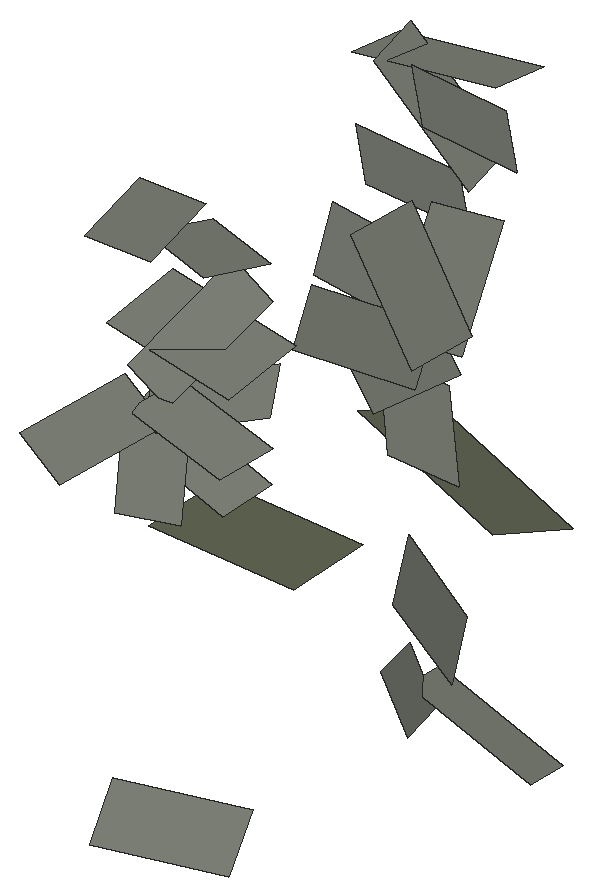
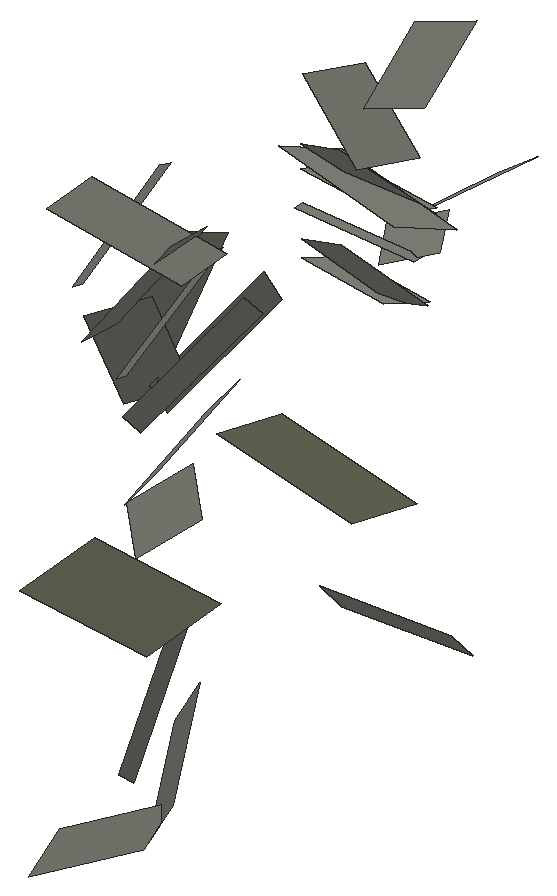
# SketchUp Ruby script. Lengths in inches.
U = 1.inch
M = Sketchup.active_model
def pt(a) = Geom::Point3d.new(a.map { |v| v * U })
def face(e, loops, mat)
  f = e.add_face(loops[0].map { |a| pt(a) })
  loops[1..].each { |l| e.add_face(l.map { |a| pt(a) }).erase! }
  f.material = f.back_material = mat if mat
  f
end
# faces: each face lists its corners as indices into pts; further lists are holes
def faces(e, pts, list, mat = nil) = list.each { |f| face(e, (f[0].is_a?(Array) ? f : [f]).map { |l| l.map { |i| pts[i] } }, mat) }
# xy, xz, yz: faces in a plane at the given z, y or x. An outline is a flat list of corners, or four numbers for a rectangle; further outlines are holes
def ring(l) = l.size == 4 ? [[l[0], l[1]], [l[2], l[1]], [l[2], l[3]], [l[0], l[3]]] : l.each_slice(2).to_a
def flat(e, list, mat, &to3) = list.each { |f| face(e, (f[0].is_a?(Array) ? f : [f]).map { |l| ring(l).map { |u, v| to3.(u, v) } }, mat) }
def xy(e, z, list, mat = nil) = flat(e, list, mat) { |x, y| [x, y, z] }
def xz(e, y, list, mat = nil) = flat(e, list, mat) { |x, z| [x, y, z] }
def yz(e, x, list, mat = nil) = flat(e, list, mat) { |y, z| [x, y, z] }
def lines(e, pts, list) = list.each { |a, b| e.add_line(pt(pts[a]), pt(pts[b])) }
# prism: a flat outline (further loops are holes) pulled along v
def prism(e, loops, v, mat = nil)
  f = face(e, loops, mat); d = Geom::Vector3d.new(v.map { |x| x * U })
  f.pushpull(f.normal.samedirection?(d) ? d.length : -d.length)
end
def box(e, o, s, mat = nil) = prism(e, [[o, [o[0] + s[0], o[1], o[2]], [o[0] + s[0], o[1] + s[1], o[2]], [o[0], o[1] + s[1], o[2]]]], [0, 0, s[2]], mat)
def at(x, y, z, deg = 0) = Geom::Transformation.translation(pt([x, y, z])) * Geom::Transformation.rotation(ORIGIN, Z_AXIS, deg.degrees)
def axes(o, x, y, z) = Geom::Transformation.new([*x, 0, *y, 0, *z, 0, *pt(o).to_a, 1])
def part(name) = M.definitions.add(name)
# library, detail: a bought-in or finely detailed component or shape, given as its bounding box
def library(name, o, s) = part(name).tap { |d| box(d.entities, o, s) }
def detail(e, o, s) = box(e.add_group.entities, o, s)
def put(e, d, t, mat = nil) = e.add_instance(d, t).tap { |i| i.material = mat if mat }
def group(e, t, mat = nil) = e.add_group.tap { |g| g.transformation = t; g.material = mat if mat }.entities
root = M.entities
M.materials.add("viburnumblaasdfas0df1w06d").color = [98, 102, 84]
M.materials.add("viburnumbladsadfasdfad0w122").color = [125, 129, 119]
c1 = part("Component\#315")
p = [[0.25,0,0],[2.05,0.01,0.35],[1.81,4.2,1.66],[0,4.19,1.3125]]
faces(c1.entities,p,[[0,1,2,3]],"viburnumbladsadfasdfad0w122")
c2 = part("viburnumblad2")
put(c2.entities,c1,axes([-19.23,-4.49,-32.18],[83.35428,0,0],[0,79.38502,0],[0,0,83.35428]))
c3 = part("Component\#314")
p = [[0.14,0,0],[2.58,0.05,0.25],[2.44,5.11,2.64],[0,5.05,2.39]]
faces(c3.entities,p,[[0,1,2,3]],"viburnumblaasdfas0df1w06d")
c4 = part("viburnumblad1\#2")
put(c4.entities,c3,axes([-37.25,6.23,19.31],[75.98784,0,0],[0,65.50676,0],[0,0,75.98784]))
put(root,c2,axes([1241.59,200.74,28.69],[-0.01126,-0.00309,0.00036],[0.00297,-0.01108,-0.00222],[0.00093,-0.00205,0.01147]))
put(root,c2,axes([1240.14,199.86,22.73],[0.01011,-0.00136,-0.00516],[0.0034,0.00814,0.00428],[0.00337,-0.00599,0.00744]))
put(root,c2,axes([1243,209.77,25.51],[-0.00283,0.01146,0.00038],[-0.0094,-0.00257,0.00741],[0.00704,0.00146,0.00821]))
put(root,c2,axes([1242.51,198.01,23.72],[-0.00968,0.00131,0.00494],[-0.00285,-0.01022,-0.00281],[0.00419,-0.00363,0.00837]))
put(root,c4,axes([1238.92,204.09,17.79],[-0.00228,-0.0125,-0.00287],[0.01428,-0.00152,-0.00471],[0.00336,-0.00314,0.01093]))
put(root,c2,axes([1242.72,210.15,24.1],[-0.00853,0.00601,0.00433],[-0.00446,-0.01051,0.00545],[0.00645,0.00235,0.00846]))
put(root,c2,axes([1243.16,208.5,21.67],[-0.00501,0.0098,0.00679],[-0.00808,-0.00821,0.00589],[0.00877,-0.00196,0.0093]))
put(root,c2,axes([1239.68,211.03,28.49],[-0.00073,-0.01199,-0.00108],[0.01339,-0.00063,-0.00213],[0.0019,-0.00123,0.01236]))
put(root,c2,axes([1240.09,198.93,12.3],[0.00083,-0.00664,-0.00958],[0.01085,0.00394,-0.00179],[0.00425,-0.00877,0.00644]))
put(root,c2,axes([1241.86,210.07,10.17],[-0.00779,-0.00011,0.00854],[0.00262,-0.01208,0.00224],[0.0089,0.00345,0.00816]))
put(root,c2,axes([1242.76,209.72,20.15],[-0.00997,0.00134,0.00814],[-0.00176,-0.01174,-0.00023],[0.00802,-0.0014,0.01005]))
put(root,c2,axes([1240.92,201.87,27.55],[-0.00596,-0.00978,-0.00229],[0.01005,-0.00579,-0.00143],[0.00006,-0.0027,0.01137]))
put(root,c2,axes([1240.07,201.3,25.98],[-0.00385,-0.0119,-0.00772],[0.01402,-0.00199,-0.00394],[0.00214,-0.0084,0.01187]))
put(root,c2,axes([1241.78,210.5,19.18],[-0.00949,-0.00826,0.00492],[0.00532,-0.00908,-0.00498],[0.00706,-0.00173,0.0107]))
put(root,c2,axes([1240.91,198.53,24.71],[0.00968,-0.00131,-0.00494],[0.00378,0.00904,0.00475],[0.00337,-0.00599,0.00744]))
put(root,c2,axes([1242.85,209.46,11.4],[-0.00627,0.00896,0.00619],[-0.00305,-0.00837,0.00903],[0.01046,0.00298,0.00629]))
put(root,c2,axes([1242.19,199.42,23.07],[-0.0092,-0.00594,0.0008],[0.00497,-0.0084,-0.00522],[0.00323,-0.00386,0.00866]))
put(root,c4,axes([1239.6,211.76,17],[-0.00406,-0.01328,0.00293],[0.01275,-0.00581,-0.00863],[0.008,0.00014,0.01172]))
put(root,c2,axes([1240.8125,199.62,23.74],[0.00449,-0.00779,-0.00619],[0.00881,0.00487,0.00016],[0.00266,-0.00553,0.00801]))
put(root,c2,axes([1241.22,200.35,22.63],[-0.00331,-0.00841,-0.00433],[0.01007,-0.00189,-0.00393],[0.00222,-0.00567,0.00805]))
put(root,c2,axes([1243.68,206.72,21.22],[-0.00309,0.00736,0.0079],[-0.00654,-0.00921,0.0057],[0.00929,-0.00262,0.00521]))
put(root,c2,axes([1241.17,211.13,10.67],[0.00148,-0.01296,0.00142],[0.00776,-0.00002,-0.00823],[0.00903,0.00196,0.00851]))
put(root,c2,axes([1244.27,210.09,26.35],[-0.00889,0.00626,0.00451],[-0.00413,-0.00973,0.00504],[0.00645,0.00235,0.00846]))
put(root,c2,axes([1242.8125,206.79,22.42],[0.00746,0.0085,-0.0048],[-0.00195,0.00645,0.00799],[0.00881,-0.00455,0.00477]))
put(root,c2,axes([1242.15,199.1,24.48],[-0.00334,-0.0097,-0.00381],[0.01007,-0.00189,-0.00393],[0.0026,-0.00465,0.00851]))
put(root,c2,axes([1244.22,205.89,22.33],[0.00278,0.01118,0.00257],[-0.00655,-0.00082,0.0102],[0.00931,-0.00357,0.00467]))
